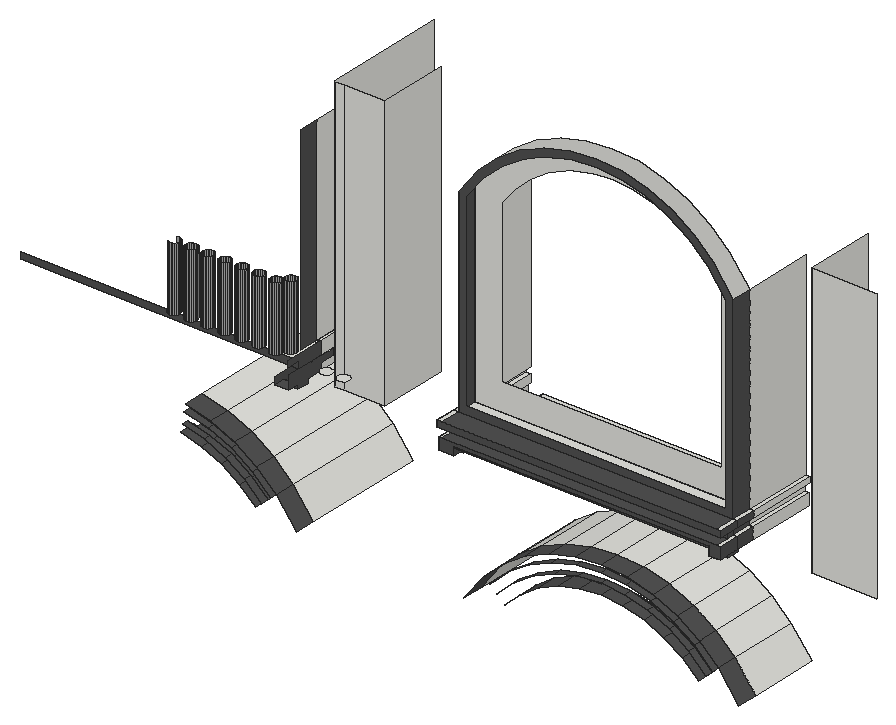
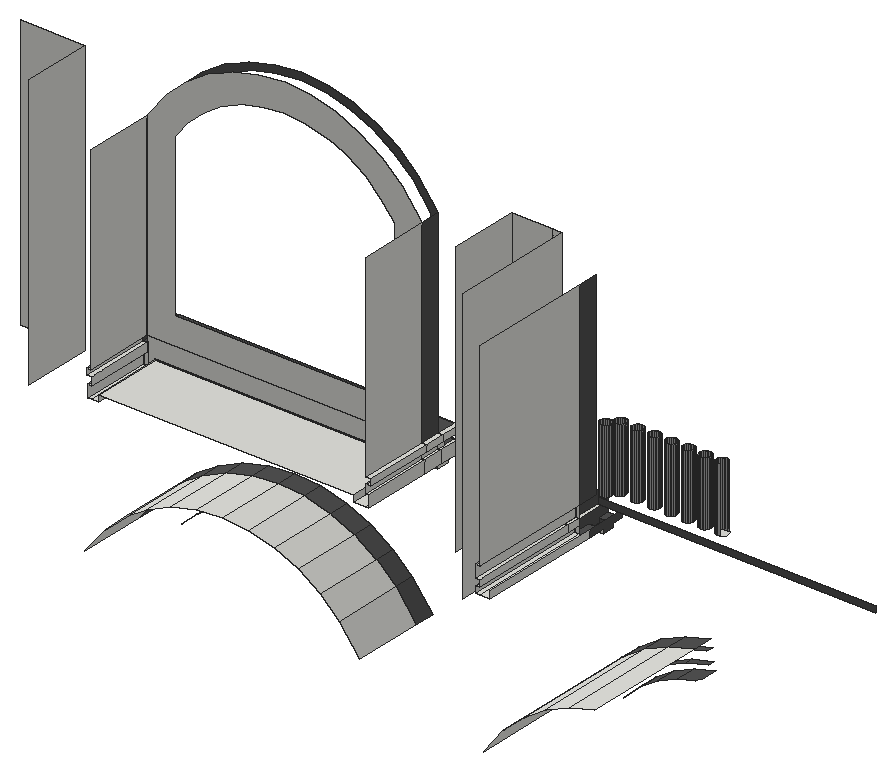
# SketchUp Ruby script. Lengths in inches.
U = 1.inch
M = Sketchup.active_model
def pt(a) = Geom::Point3d.new(a.map { |v| v * U })
def face(e, loops, mat)
  f = e.add_face(loops[0].map { |a| pt(a) })
  loops[1..].each { |l| e.add_face(l.map { |a| pt(a) }).erase! }
  f.material = f.back_material = mat if mat
  f
end
# faces: each face lists its corners as indices into pts; further lists are holes
def faces(e, pts, list, mat = nil) = list.each { |f| face(e, (f[0].is_a?(Array) ? f : [f]).map { |l| l.map { |i| pts[i] } }, mat) }
# xy, xz, yz: faces in a plane at the given z, y or x. An outline is a flat list of corners, or four numbers for a rectangle; further outlines are holes
def ring(l) = l.size == 4 ? [[l[0], l[1]], [l[2], l[1]], [l[2], l[3]], [l[0], l[3]]] : l.each_slice(2).to_a
def flat(e, list, mat, &to3) = list.each { |f| face(e, (f[0].is_a?(Array) ? f : [f]).map { |l| ring(l).map { |u, v| to3.(u, v) } }, mat) }
def xy(e, z, list, mat = nil) = flat(e, list, mat) { |x, y| [x, y, z] }
def xz(e, y, list, mat = nil) = flat(e, list, mat) { |x, z| [x, y, z] }
def yz(e, x, list, mat = nil) = flat(e, list, mat) { |y, z| [x, y, z] }
def lines(e, pts, list) = list.each { |a, b| e.add_line(pt(pts[a]), pt(pts[b])) }
# prism: a flat outline (further loops are holes) pulled along v
def prism(e, loops, v, mat = nil)
  f = face(e, loops, mat); d = Geom::Vector3d.new(v.map { |x| x * U })
  f.pushpull(f.normal.samedirection?(d) ? d.length : -d.length)
end
def box(e, o, s, mat = nil) = prism(e, [[o, [o[0] + s[0], o[1], o[2]], [o[0] + s[0], o[1] + s[1], o[2]], [o[0], o[1] + s[1], o[2]]]], [0, 0, s[2]], mat)
def at(x, y, z, deg = 0) = Geom::Transformation.translation(pt([x, y, z])) * Geom::Transformation.rotation(ORIGIN, Z_AXIS, deg.degrees)
def axes(o, x, y, z) = Geom::Transformation.new([*x, 0, *y, 0, *z, 0, *pt(o).to_a, 1])
def part(name) = M.definitions.add(name)
# library, detail: a bought-in or finely detailed component or shape, given as its bounding box
def library(name, o, s) = part(name).tap { |d| box(d.entities, o, s) }
def detail(e, o, s) = box(e.add_group.entities, o, s)
def put(e, d, t, mat = nil) = e.add_instance(d, t).tap { |i| i.material = mat if mat }
def group(e, t, mat = nil) = e.add_group.tap { |g| g.transformation = t; g.material = mat if mat }.entities
root = M.entities
M.materials.add("[0132_LightGray]").color = [169, 169, 169]
M.materials.add("[0135_DarkGray]").color = [81, 81, 81]
xy(root,482.35,[[358.5,36.95,364.76,42.1]],"[0135_DarkGray]")
xy(root,482.85,[[430.82,37.17,437.43,42.74]],"[0135_DarkGray]")
xy(root,483.16,[[549.38,35.78,554.39,41.4]],"[0135_DarkGray]")
xy(root,484.03,[[549.38,35.78,552.7,40.6875],[552.7,35.78,554.39,40.6875],[430.82,37.17,432.14,40.6875],[432.14,37.17,437.43,40.6875],[430.82,40.6875,432.14,42.74],
  [432.14,40.6875,437.43,42.74],[549.38,40.6875,552.7,41.4],[552.7,40.6875,554.39,41.4],[430.82,49.6875,432.14,80.4375],[432.14,49.6875,437.43,80.4375],
  [549.38,49.6875,552.7,80.4375],[552.7,49.6875,554.39,80.4375]])
xy(root,484.03,[[430.82,31.6875,432.14,37.17],[432.14,31.6875,437.43,37.17],[549.38,31.6875,552.7,35.78],[552.7,31.6875,554.39,35.78],[549.38,41.4,552.7,49.6875],
  [552.7,41.4,554.39,49.6875],[430.82,42.74,432.14,49.6875],[432.14,42.74,437.43,49.6875]],"[0135_DarkGray]")
xy(root,484.28,[[358.5,49.6875,363.14,104.375],[363.14,49.6875,364.76,104.375]])
xy(root,484.28,[[358.5,31.6875,364.76,36.95],[358.5,42.1,364.76,49.6875]],"[0135_DarkGray]")
xy(root,487.03,[[437.43,49.6875,549.38,80.4375]])
xy(root,487.03,[[437.43,31.6875,549.38,49.6875]],"[0135_DarkGray]")
xy(root,487.28,[[363.14,49.6875,364.76,55.75],[363.14,55.75,364.76,104.375]])
xy(root,487.72,[[437.43,31.6875,549.38,49.6875]])
xy(root,489.3125,[[430.82,31.6875,432.14,40.6875],[552.7,31.6875,554.39,40.6875],[430.82,40.6875,432.14,49.6875],[552.7,40.6875,554.39,49.6875],[430.82,49.6875,432.14,80.4375],
  [552.7,49.6875,554.39,80.4375]])
xy(root,489.3125,[[432.14,31.6875,552.7,37.6875]],"[0135_DarkGray]")
xy(root,490.18,[[363.14,37.6875,364.64,49.6875],[364.64,37.6875,364.76,55.75],[363.14,49.6875,364.64,55.75],[363.14,55.75,364.64,104.375]])
xy(root,492.99,[[430.01,49.6875,432.14,80.4375],[552.7,49.6875,554.64,80.4375]])
xy(root,492.99,[[430.01,31.6875,432.14,40.6875],[432.14,31.6875,552.7,37.6875],[552.7,31.6875,554.64,40.6875],[430.01,40.6875,432.14,49.6875],[552.7,40.6875,554.64,49.6875]],"[0135_DarkGray]")
xy(root,495.66,[[430.01,31.6875,432.14,40.6875],[552.82,31.6875,554.64,40.6875],[312.48,31.88,311.85,31.96,311.26,32.21,310.75,32.6,310.37,33.1,310.12,33.6875,310.04,34.32,310.12,34.95,310.37,35.54,310.75,36.04,311.26,36.43,311.85,36.67,312.48,36.76,313.11,36.67,313.7,36.43,314.2,36.04,314.59,35.54,314.83,34.95,314.91,34.32,314.83,33.6875,314.59,33.1,314.2,32.6,313.7,32.21,313.11,31.96],[319.91,31.88,319.28,31.96,318.7,32.21,318.19,32.6,317.8,33.1,317.56,33.6875,317.48,34.32,317.56,34.95,317.8,35.54,318.19,36.04,318.7,36.43,319.28,36.67,319.91,36.76,320.54,36.67,321.13,36.43,321.64,36.04,322.03,35.54,322.27,34.95,322.35,34.32,322.27,33.6875,322.03,33.1,321.64,32.6,321.13,32.21,320.54,31.96],[327.35,31.88,326.72,31.96,326.13,32.21,325.63,32.6,325.24,33.1,325,33.6875,324.91,34.32,325,34.95,325.24,35.54,325.63,36.04,326.13,36.43,326.72,36.67,327.35,36.76,327.98,36.67,328.57,36.43,329.08,36.04,329.46,35.54,329.71,34.95,329.79,34.32,329.71,33.6875,329.46,33.1,329.08,32.6,328.57,32.21,327.98,31.96],
  [334.79,31.88,334.16,31.96,333.57,32.21,333.07,32.6,332.68,33.1,332.43,33.6875,332.35,34.32,332.43,34.95,332.68,35.54,333.07,36.04,333.57,36.43,334.16,36.67,334.79,36.76,335.42,36.67,336.01,36.43,336.51,36.04,336.9,35.54,337.14,34.95,337.23,34.32,337.14,33.6875,336.9,33.1,336.51,32.6,336.01,32.21,335.42,31.96],[342.23,31.88,341.6,31.96,341.01,32.21,340.5,32.6,340.12,33.1,339.87,33.6875,339.79,34.32,339.87,34.95,340.12,35.54,340.5,36.04,341.01,36.43,341.6,36.67,342.23,36.76,342.86,36.67,343.45,36.43,343.95,36.04,344.34,35.54,344.58,34.95,344.66,34.32,344.58,33.6875,344.34,33.1,343.95,32.6,343.45,32.21,342.86,31.96],[349.66,31.88,349.03,31.96,348.45,32.21,347.94,32.6,347.55,33.1,347.31,33.6875,347.23,34.32,347.31,34.95,347.55,35.54,347.94,36.04,348.45,36.43,349.03,36.67,349.66,36.76,350.29,36.67,350.88,36.43,351.39,36.04,351.78,35.54,352.02,34.95,352.1,34.32,352.02,33.6875,351.78,33.1,351.39,32.6,350.88,32.21,350.29,31.96],[357.1,31.88,356.47,31.96,355.88,32.21,355.38,32.6,354.99,33.1,354.75,33.6875,354.66,34.32,354.75,34.95,354.99,35.54,355.38,36.04,355.88,36.43,356.47,36.67,357.1,36.76,357.73,36.67,358.32,36.43,358.83,36.04,359.21,35.54,359.46,34.95,359.54,34.32,359.46,33.6875,359.21,33.1,358.83,32.6,358.32,32.21,357.73,31.96],[379.41,31.88,380.04,31.96,380.63,32.21,381.14,32.6,381.53,33.1,381.77,33.6875,381.85,34.32,381.77,34.95,381.53,35.54,381.14,36.04,380.63,36.43,380.04,36.67,379.41,36.76,378.78,36.67,378.2,36.43,377.69,36.04,377.3,35.54,377.06,34.95,376.98,34.32,377.06,33.6875,377.3,33.1,377.69,32.6,378.2,32.21,378.78,31.96],
  [386.85,31.88,387.48,31.96,388.07,32.21,388.58,32.6,388.96,33.1,389.21,33.6875,389.29,34.32,389.21,34.95,388.96,35.54,388.58,36.04,388.07,36.43,387.48,36.67,386.85,36.76,386.22,36.67,385.63,36.43,385.13,36.04,384.74,35.54,384.5,34.95,384.41,34.32,384.5,33.6875,384.74,33.1,385.13,32.6,385.63,32.21,386.22,31.96],[360.59,35.72,359.96,35.81,359.37,36.05,358.86,36.4375,358.48,36.94,358.23,37.53,358.15,38.16,358.23,38.79,358.48,39.38,358.86,39.89,359.37,40.27,359.96,40.52,360.59,40.6,361.22,40.52,361.8,40.27,362.31,39.89,362.7,39.38,362.94,38.79,363.02,38.16,362.94,37.53,362.7,36.94,362.31,36.4375,361.8,36.05,361.22,35.81],[430.01,40.6875,432.14,49.6875],[432.14,40.6875,552.7,49.6875],[552.7,40.6875,552.82,49.6875],
  [552.82,40.6875,554.64,49.6875],[362.82,49.6875,363.14,104.375],[363.14,49.6875,364.64,104.375],[430.01,49.6875,432.14,80.4375],[552.82,49.6875,554.64,80.4375]])
xy(root,495.66,[[432.14,31.6875,552.82,40.6875]],"[0135_DarkGray]")
xz(root,31.6875,[[430.82,484.03,437.43,484.03,437.43,487.72,549.38,487.72,549.38,484.03,554.39,484.03,554.39,489.3125,430.82,489.3125],[437.43,487.03,549.38,487.72],[430.01,492.99,554.64,495.66]],"[0135_DarkGray]")
xz(root,35.78,[[549.38,483.16,554.39,484.03]],"[0135_DarkGray]")
xz(root,36.95,[[358.5,482.35,364.76,484.28]],"[0135_DarkGray]")
xz(root,37.17,[[430.82,482.85,437.43,484.03]],"[0135_DarkGray]")
xz(root,37.6875,[[432.14,489.3125,552.7,492.99],[242.14,490.18,364.64,493.07]],"[0135_DarkGray]")
xz(root,40.6875,[[[432.14,495.66,552.82,495.66,552.82,582.07,543.9,593.68,535.43,601.54,525.77,607.9,518.81,610.98,515.2,612.57,504,615.43,492.48,616.39,480.96,615.43,469.76,612.57,466.15,610.98,459.18,607.9,449.53,601.54,441.0625,593.68,432.14,582.07],[435.27,498.79,435.27,581.01,443.38,591.5625,451.47,599.07,460.6875,605.14,467.41,608.11,470.78,609.6,481.48,612.33,492.48,613.25,503.48,612.33,514.17,609.6,517.54,608.11,524.27,605.14,533.49,599.07,541.57,591.5625,549.69,581.01,549.69,498.79]]],"[0135_DarkGray]")
xz(root,41.4,[[549.38,483.16,554.39,484.03]])
xz(root,42.1,[[358.5,482.35,364.76,484.28]])
xz(root,42.74,[[430.82,482.85,437.43,484.03]],"[0135_DarkGray]")
xz(root,49.6875,[[370.55,480,370.74,600],[370.74,480,374.55,600],[374.55,480,392.7,600],[580.01,480,608.5,600],[430.82,484.03,432.14,489.3125],
  [432.14,484.03,437.43,484.03,437.43,487.72,549.38,487.72,549.38,484.03,552.7,484.03,552.7,495.66,432.14,495.66],[552.7,484.03,554.39,489.3125],[363.14,484.28,364.76,487.28],[437.43,487.03,549.38,487.72],[363.14,490.18,364.64,495.66],
  [[432.14,495.66,432.14,582.07,441.0625,593.68,449.53,601.54,459.18,607.9,466.15,610.98,469.76,612.57,480.96,615.43,492.48,616.39,504,615.43,515.2,612.57,518.81,610.98,525.77,607.9,535.43,601.54,543.9,593.68,552.82,582.07,552.82,495.66],[444.14,507.66,540.82,507.66,540.82,577.99,534.99,585.57,527.99,592.07,520.01,597.33,513.96,600,511.27,601.19,502,603.55,492.48,604.35,489.7,604.11,483.7,603.61,482.95,603.55,473.69,601.19,471,600,464.95,597.33,456.97,592.07,449.96,585.57,444.14,577.99]]])
xz(root,55.75,[[363.14,487.28,364.76,490.18]])
yz(root,358.5,[[49.6875,484.28,104.375,487.28]])
yz(root,358.5,[[36.95,482.35,36.95,484.28,31.6875,484.28,31.6875,487.28,49.6875,487.28,49.6875,484.28,42.1,484.28,42.1,482.35]],"[0135_DarkGray]")
yz(root,362.82,[[49.6875,495.66,104.375,582.07]])
yz(root,362.82,[[40.6875,495.66,49.6875,582.07]],"[0135_DarkGray]")
yz(root,363.14,[[49.6875,487.28,55.75,490.18],[55.75,487.28,104.375,490.18]])
yz(root,364.64,[[49.6875,490.18,104.375,495.66]])
yz(root,364.64,[[37.6875,490.18,49.6875,490.18,49.6875,495.66,31.6875,495.66,31.6875,493.07,37.6875,493.07]],"[0135_DarkGray]")
yz(root,364.76,[[49.6875,484.28,104.375,487.28]])
yz(root,364.76,[[36.95,482.35,42.1,482.35,42.1,484.28,49.6875,484.28,49.6875,487.28,55.75,487.28,55.75,490.18,31.6875,490.18,31.6875,484.28,36.95,484.28]],"[0135_DarkGray]")
yz(root,370.55,[[49.6875,480,104.375,600]])
yz(root,392.7,[[49.6875,480,80.4375,600]])
yz(root,430.01,[[31.6875,492.99,40.6875,495.66],[40.6875,492.99,49.6875,495.66],[49.6875,492.99,80.4375,495.66]])
yz(root,430.82,[[37.17,482.85,42.74,484.03],[31.6875,484.03,40.6875,489.3125],[40.6875,484.03,49.6875,489.3125],[49.6875,484.03,80.4375,489.3125]])
yz(root,432.14,[[37.6875,489.3125,40.6875,492.99],[40.6875,489.3125,49.6875,492.99],[49.6875,489.3125,80.4375,492.99],[49.6875,495.66,80.4375,582.07]])
yz(root,432.14,[[40.6875,495.66,49.6875,582.07]],"[0135_DarkGray]")
yz(root,437.43,[[49.6875,484.03,80.4375,487.03],[31.6875,487.03,40.6875,487.72],[40.6875,487.03,49.6875,487.72]])
yz(root,437.43,[[37.17,482.85,42.74,484.03],[31.6875,484.03,40.6875,487.03],[40.6875,484.03,49.6875,487.03]],"[0135_DarkGray]")
yz(root,549.38,[[49.6875,484.03,80.4375,487.03],[31.6875,487.03,40.6875,487.72],[40.6875,487.03,49.6875,487.72]])
yz(root,549.38,[[35.78,483.16,41.4,484.03],[31.6875,484.03,40.6875,487.03],[40.6875,484.03,49.6875,487.03]],"[0135_DarkGray]")
yz(root,552.7,[[49.6875,489.3125,80.4375,492.99]])
yz(root,552.7,[[37.6875,489.3125,40.6875,492.99],[40.6875,489.3125,49.6875,492.99]],"[0135_DarkGray]")
yz(root,552.82,[[49.6875,495.66,80.4375,582.07]])
yz(root,552.82,[[40.6875,495.66,49.6875,582.07]],"[0135_DarkGray]")
yz(root,554.39,[[49.6875,484.03,80.4375,489.3125]])
yz(root,554.39,[[35.78,483.16,41.4,484.03],[31.6875,484.03,40.6875,489.3125],[40.6875,484.03,49.6875,489.3125]],"[0135_DarkGray]")
yz(root,554.64,[[49.6875,492.99,80.4375,495.66]])
yz(root,554.64,[[31.6875,492.99,40.6875,495.66],[40.6875,492.99,49.6875,495.66]],"[0135_DarkGray]")
yz(root,580.01,[[49.6875,480,80.4375,600]])
p = [[361.14,49.6875,423.26],[352.21,49.6875,434.86],[352.21,40.6875,434.86],[361.14,40.6875,423.26],[434.7,49.6875,423.26],[443.625,49.6875,434.86],
  [443.625,40.6875,434.86],[434.7,40.6875,423.26],[546.46,49.6875,434.86],[555.39,49.6875,423.26],[555.39,40.6875,423.26],[546.46,40.6875,434.86],
  [352.21,104.375,434.86],[361.14,104.375,423.26],[434.7,80.4375,423.26],[443.625,80.4375,434.86],[546.46,80.4375,434.86],[555.39,80.4375,423.26],
  [336.3,49.6875,433.26],[343.31,49.6875,426.75],[343.31,40.6875,426.75],[336.3,40.6875,433.26],[452.53,49.6875,426.75],[459.53,49.6875,433.26],
  [459.53,40.6875,433.26],[452.53,40.6875,426.75],[530.55,49.6875,433.26],[537.56,49.6875,426.75],[537.56,40.6875,426.75],[530.55,40.6875,433.26],
  [345.9375,43.6875,429.15],[338.5,43.6875,436.06],[338.5,40.6875,436.06],[345.9375,40.6875,429.15],[456.63,43.6875,436.95],[449.06,43.6875,429.91],
  [449.06,40.6875,429.91],[456.63,40.6875,436.95],[541.02,43.6875,429.91],[533.45,43.6875,436.95],[533.45,40.6875,436.95],[541.02,40.6875,429.91],
  [341.7,43.6875,440.13],[349.77,43.6875,432.64],[349.77,40.6875,432.64],[341.7,40.6875,440.13],[445.98,43.6875,432.71],[454.0625,43.6875,440.22],
  [454.0625,40.6875,440.22],[445.98,40.6875,432.71],[536.02,43.6875,440.22],[544.1,43.6875,432.71],[544.1,40.6875,432.71],[536.02,40.6875,440.22],
  [328.32,49.6875,438.52],[328.32,40.6875,438.52],[467.51,49.6875,438.52],[467.51,40.6875,438.52],[522.57,49.6875,438.52],[522.57,40.6875,438.52],
  [343.74,49.6875,442.73],[343.74,40.6875,442.73],[452.09,49.6875,442.73],[452.09,40.6875,442.73],[537.99,49.6875,442.73],[537.99,40.6875,442.73],
  [343.74,104.375,442.73],[452.09,80.4375,442.73],[537.99,80.4375,442.73],[330.02,43.6875,441.64],[330.02,40.6875,441.64],[465.27,43.6875,442.63],
  [465.27,40.6875,442.63],[524.82,43.6875,442.63],[524.82,40.6875,442.63],[319.58,49.6875,442.38],[319.58,40.6875,442.38],[476.25,49.6875,442.38],
  [476.25,40.6875,442.38],[513.83,49.6875,442.38],[513.83,40.6875,442.38],[332.51,43.6875,446.1875],[332.51,40.6875,446.1875],[463.27,43.6875,446.29],
  [463.27,40.6875,446.29],[526.81,43.6875,446.29],[526.81,40.6875,446.29],[320.74,43.6875,445.74],[320.74,40.6875,445.74],[310.32,40.6875,444.74],
  [310.32,47.6875,444.74],[311.64,47.6875,444.4],[311.64,49.6875,444.4],[483.7,49.6875,444.27],[483.7,47.6875,444.27],[485.52,47.6875,444.74],
  [485.52,40.6875,444.74],[504.57,49.6875,444.74],[504.57,40.6875,444.74],[474.72,43.6875,446.81],[474.72,40.6875,446.81],[515.36,43.6875,446.81],
  [515.36,40.6875,446.81],[334.09,49.6875,449.09],[334.09,40.6875,449.09],[461.75,49.6875,449.09],[461.75,40.6875,449.09],[528.34,49.6875,449.09],
  [528.34,40.6875,449.09],[334.09,104.375,449.09],[461.75,80.4375,449.09],[528.34,80.4375,449.09],[485.52,49.6875,444.74],[489.7,47.6875,445.09],
  [489.7,49.6875,445.09],[495.04,49.6875,445.53],[495.04,40.6875,445.53],[310.91,43.6875,448.25],[310.91,40.6875,448.25],[322.43,43.6875,450.64],
  [322.43,40.6875,450.64],[473.36,43.6875,450.74],[473.36,40.6875,450.74],[516.72,43.6875,450.74],[516.72,40.6875,450.74],[484.74,43.6875,449.36],
  [484.74,40.6875,449.36],[505.34,43.6875,449.36],[505.34,40.6875,449.36],[323.51,49.6875,453.76],[323.51,40.6875,453.76],[472.32,49.6875,453.76],
  [472.32,40.6875,453.76],[517.76,49.6875,453.76],[517.76,40.6875,453.76],[323.51,104.375,453.76],[472.32,80.4375,453.76],[517.76,80.4375,453.76],
  [495.04,43.6875,450.22],[495.04,40.6875,450.22],[311.76,43.6875,453.36],[311.76,40.6875,453.36],[484.05,43.6875,453.47],[484.05,40.6875,453.47],
  [506.03,43.6875,453.47],[506.03,40.6875,453.47],[495.04,43.6875,454.38],[495.04,40.6875,454.38],[312.3125,49.6875,456.61],[312.3125,40.6875,456.61],
  [483.52,49.6875,456.61],[483.52,40.6875,456.61],[506.5625,49.6875,456.61],[506.5625,40.6875,456.61],[312.3125,104.375,456.61],[483.52,80.4375,456.61],
  [506.5625,80.4375,456.61],[495.04,49.6875,457.57],[495.04,40.6875,457.57],[495.04,80.4375,457.57],[311.85,31.96,495.66],[312.48,31.88,495.66],
  [312.48,31.88,523.91],[311.85,31.96,523.91],[313.11,31.96,495.66],[313.11,31.96,523.91],[319.28,31.96,495.66],[319.91,31.88,495.66],
  [319.91,31.88,523.91],[319.28,31.96,523.91],[320.54,31.96,495.66],[320.54,31.96,523.91],[326.72,31.96,495.66],[327.35,31.88,495.66],
  [327.35,31.88,523.91],[326.72,31.96,523.91],[327.98,31.96,495.66],[327.98,31.96,523.91],[334.16,31.96,495.66],[334.79,31.88,495.66],
  [334.79,31.88,523.91],[334.16,31.96,523.91],[335.42,31.96,495.66],[335.42,31.96,523.91],[341.6,31.96,495.66],[342.23,31.88,495.66],
  [342.23,31.88,523.91],[341.6,31.96,523.91],[342.86,31.96,495.66],[342.86,31.96,523.91],[349.03,31.96,495.66],[349.66,31.88,495.66],
  [349.66,31.88,523.91],[349.03,31.96,523.91],[350.29,31.96,495.66],[350.29,31.96,523.91],[356.47,31.96,495.66],[357.1,31.88,495.66],
  [357.1,31.88,523.91],[356.47,31.96,523.91],[357.73,31.96,495.66],[357.73,31.96,523.91],[311.26,32.21,495.66],[311.26,32.21,523.91],
  [313.7,32.21,495.66],[313.7,32.21,523.91],[318.7,32.21,495.66],[318.7,32.21,523.91],[321.13,32.21,495.66],[321.13,32.21,523.91],
  [326.13,32.21,495.66],[326.13,32.21,523.91],[328.57,32.21,495.66],[328.57,32.21,523.91],[333.57,32.21,495.66],[333.57,32.21,523.91],
  [336.01,32.21,495.66],[336.01,32.21,523.91],[341.01,32.21,495.66],[341.01,32.21,523.91],[343.45,32.21,495.66],[343.45,32.21,523.91],
  [348.45,32.21,495.66],[348.45,32.21,523.91],[350.88,32.21,495.66],[350.88,32.21,523.91],[355.88,32.21,495.66],[355.88,32.21,523.91],
  [358.32,32.21,495.66],[358.32,32.21,523.91],[314.2,32.6,495.66],[314.2,32.6,523.91],[318.19,32.6,495.66],[318.19,32.6,523.91],
  [321.64,32.6,495.66],[321.64,32.6,523.91],[325.63,32.6,495.66],[325.63,32.6,523.91],[329.08,32.6,495.66],[329.08,32.6,523.91],
  [333.07,32.6,495.66],[333.07,32.6,523.91],[336.51,32.6,495.66],[336.51,32.6,523.91],[340.5,32.6,495.66],[340.5,32.6,523.91],
  [343.95,32.6,495.66],[343.95,32.6,523.91],[347.94,32.6,495.66],[347.94,32.6,523.91],[351.39,32.6,495.66],[351.39,32.6,523.91],
  [355.38,32.6,495.66],[355.38,32.6,523.91],[358.83,32.6,495.66],[358.83,32.6,523.91],[314.59,33.1,495.66],[314.59,33.1,523.91],
  [317.8,33.1,495.66],[317.8,33.1,523.91],[322.03,33.1,495.66],[322.03,33.1,523.91],[325.24,33.1,495.66],[325.24,33.1,523.91],
  [329.46,33.1,495.66],[329.46,33.1,523.91],[332.68,33.1,495.66],[332.68,33.1,523.91],[336.9,33.1,495.66],[336.9,33.1,523.91],
  [340.12,33.1,495.66],[340.12,33.1,523.91],[344.34,33.1,495.66],[344.34,33.1,523.91],[347.55,33.1,495.66],[347.55,33.1,523.91],
  [351.78,33.1,495.66],[351.78,33.1,523.91],[354.99,33.1,495.66],[354.99,33.1,523.91],[359.21,33.1,495.66],[359.21,33.1,523.91],
  [314.83,33.6875,495.66],[314.83,33.6875,523.91],[317.56,33.6875,495.66],[317.56,33.6875,523.91],[322.27,33.6875,495.66],[322.27,33.6875,523.91],
  [325,33.6875,495.66],[325,33.6875,523.91],[329.71,33.6875,495.66],[329.71,33.6875,523.91],[332.43,33.6875,495.66],[332.43,33.6875,523.91],
  [337.14,33.6875,495.66],[337.14,33.6875,523.91],[339.87,33.6875,495.66],[339.87,33.6875,523.91],[344.58,33.6875,495.66],[344.58,33.6875,523.91],
  [347.31,33.6875,495.66],[347.31,33.6875,523.91],[352.02,33.6875,495.66],[352.02,33.6875,523.91],[354.75,33.6875,495.66],[354.75,33.6875,523.91],
  [359.46,33.6875,495.66],[359.46,33.6875,523.91],[314.91,34.32,495.66],[314.91,34.32,523.91],[317.48,34.32,495.66],[317.48,34.32,523.91],
  [322.35,34.32,495.66],[322.35,34.32,523.91],[324.91,34.32,495.66],[324.91,34.32,523.91],[329.79,34.32,495.66],[329.79,34.32,523.91],
  [332.35,34.32,495.66],[332.35,34.32,523.91],[337.23,34.32,495.66],[337.23,34.32,523.91],[339.79,34.32,495.66],[339.79,34.32,523.91],
  [344.66,34.32,495.66],[344.66,34.32,523.91],[347.23,34.32,495.66],[347.23,34.32,523.91],[352.1,34.32,495.66],[352.1,34.32,523.91],
  [354.66,34.32,495.66],[354.66,34.32,523.91],[359.54,34.32,495.66],[359.54,34.32,523.91],[314.83,34.95,495.66],[314.83,34.95,523.91],
  [317.56,34.95,495.66],[317.56,34.95,523.91],[322.27,34.95,495.66],[322.27,34.95,523.91],[325,34.95,495.66],[325,34.95,523.91],
  [329.71,34.95,495.66],[329.71,34.95,523.91],[332.43,34.95,495.66],[332.43,34.95,523.91],[337.14,34.95,495.66],[337.14,34.95,523.91],
  [339.87,34.95,495.66],[339.87,34.95,523.91],[344.58,34.95,495.66],[344.58,34.95,523.91],[347.31,34.95,495.66],[347.31,34.95,523.91],
  [352.02,34.95,495.66],[352.02,34.95,523.91],[354.75,34.95,495.66],[354.75,34.95,523.91],[359.46,34.95,495.66],[359.46,34.95,523.91],
  [314.59,35.54,495.66],[314.59,35.54,523.91],[317.8,35.54,495.66],[317.8,35.54,523.91],[322.03,35.54,495.66],[322.03,35.54,523.91],
  [325.24,35.54,495.66],[325.24,35.54,523.91],[329.46,35.54,495.66],[329.46,35.54,523.91],[332.68,35.54,495.66],[332.68,35.54,523.91],
  [336.9,35.54,495.66],[336.9,35.54,523.91],[340.12,35.54,495.66],[340.12,35.54,523.91],[344.34,35.54,495.66],[344.34,35.54,523.91],
  [347.55,35.54,495.66],[347.55,35.54,523.91],[351.78,35.54,495.66],[351.78,35.54,523.91],[354.99,35.54,495.66],[354.99,35.54,523.91],
  [359.21,35.54,495.66],[359.21,35.54,523.91],[314.2,36.04,495.66],[314.2,36.04,523.91],[318.19,36.04,495.66],[318.19,36.04,523.91],
  [321.64,36.04,495.66],[321.64,36.04,523.91],[325.63,36.04,495.66],[325.63,36.04,523.91],[329.08,36.04,495.66],[329.08,36.04,523.91],
  [333.07,36.04,495.66],[333.07,36.04,523.91],[336.51,36.04,495.66],[336.51,36.04,523.91],[340.5,36.04,495.66],[340.5,36.04,523.91],
  [343.95,36.04,495.66],[343.95,36.04,523.91],[347.94,36.04,495.66],[347.94,36.04,523.91],[351.39,36.04,495.66],[351.39,36.04,523.91],
  [355.38,36.04,495.66],[355.38,36.04,523.91],[358.83,36.04,495.66],[358.83,36.04,523.91],[359.96,35.81,495.66],[360.59,35.72,495.66],
  [360.59,35.72,523.91],[359.96,35.81,523.91],[361.22,35.81,495.66],[361.22,35.81,523.91],[359.37,36.05,495.66],[359.37,36.05,523.91],
  [361.8,36.05,495.66],[361.8,36.05,523.91],[313.7,36.43,495.66],[313.7,36.43,523.91],[318.7,36.43,495.66],[318.7,36.43,523.91],
  [321.13,36.43,495.66],[321.13,36.43,523.91],[326.13,36.43,495.66],[326.13,36.43,523.91],[328.57,36.43,495.66],[328.57,36.43,523.91],
  [333.57,36.43,495.66],[333.57,36.43,523.91],[336.01,36.43,495.66],[336.01,36.43,523.91],[341.01,36.43,495.66],[341.01,36.43,523.91],
  [343.45,36.43,495.66],[343.45,36.43,523.91],[348.45,36.43,495.66],[348.45,36.43,523.91],[350.88,36.43,495.66],[350.88,36.43,523.91],
  [355.88,36.43,495.66],[355.88,36.43,523.91],[358.32,36.43,495.66],[358.32,36.43,523.91],[358.86,36.4375,495.66],[358.86,36.4375,523.91],
  [362.31,36.4375,495.66],[362.31,36.4375,523.91],[313.11,36.67,495.66],[313.11,36.67,523.91],[319.28,36.67,495.66],[319.28,36.67,523.91],
  [320.54,36.67,495.66],[320.54,36.67,523.91],[326.72,36.67,495.66],[326.72,36.67,523.91],[327.98,36.67,495.66],[327.98,36.67,523.91],
  [334.16,36.67,495.66],[334.16,36.67,523.91],[335.42,36.67,495.66],[335.42,36.67,523.91],[341.6,36.67,495.66],[341.6,36.67,523.91],
  [342.86,36.67,495.66],[342.86,36.67,523.91],[349.03,36.67,495.66],[349.03,36.67,523.91],[350.29,36.67,495.66],[350.29,36.67,523.91],
  [356.47,36.67,495.66],[356.47,36.67,523.91],[357.73,36.67,495.66],[357.73,36.67,523.91],[358.48,36.94,495.66],[358.48,36.94,523.91],
  [362.7,36.94,495.66],[362.7,36.94,523.91],[312.48,36.76,495.66],[311.85,36.67,495.66],[311.85,36.67,523.91],[312.48,36.76,523.91],
  [319.91,36.76,495.66],[319.91,36.76,523.91],[327.35,36.76,495.66],[327.35,36.76,523.91],[334.79,36.76,495.66],[334.79,36.76,523.91],
  [342.23,36.76,495.66],[342.23,36.76,523.91],[349.66,36.76,495.66],[349.66,36.76,523.91],[357.1,36.76,495.66],[357.1,36.76,523.91],
  [358.23,37.53,495.66],[358.23,37.53,523.91],[362.94,37.53,495.66],[362.94,37.53,523.91],[358.15,38.16,495.66],[358.15,38.16,523.91],
  [363.02,38.16,495.66],[363.02,38.16,523.91],[358.23,38.79,495.66],[358.23,38.79,523.91],[362.94,38.79,495.66],[362.94,38.79,523.91],
  [358.48,39.38,495.66],[358.48,39.38,523.91],[362.7,39.38,495.66],[362.7,39.38,523.91],[358.86,39.89,495.66],[358.86,39.89,523.91],
  [362.31,39.89,495.66],[362.31,39.89,523.91],[359.37,40.27,495.66],[359.37,40.27,523.91],[361.8,40.27,495.66],[361.8,40.27,523.91],
  [359.96,40.52,495.66],[359.96,40.52,523.91],[361.22,40.52,495.66],[361.22,40.52,523.91],[360.59,40.6,495.66],[360.59,40.6,523.91],
  [363.14,37.6875,490.18],[363.14,37.6875,487.28],[432.14,37.6875,492.99],[432.14,37.6875,495.66],[432.14,37.6875,487.03],[432.14,37.6875,489.3125]]
faces(root,p,[[0,1,2,3],[4,5,6,7],[8,9,10,11],[18,19,20,21],[22,23,24,25],[26,27,28,29],[30,31,32,33],[34,35,36,37],
  [38,39,40,41],[42,43,44,45],[46,47,48,49],[50,51,52,53],[54,18,21,55],[23,56,57,24],[58,26,29,59],[1,60,61,2],
  [5,62,63,6],[64,8,11,65],[31,69,70,32],[71,34,37,72],[39,73,74,40],[75,54,55,76],[56,77,78,57],[79,58,59,80],
  [81,42,45,82],[47,83,84,48],[85,50,53,86],[69,87,88,70],[89,90,91,92,75,76],[77,93,94,95,96,78],[97,79,80,98],[99,71,72,100],
  [73,101,102,74],[60,103,104,61],[62,105,106,63],[107,64,65,108],[96,95,113,114,115,116],[115,97,98,116],[87,117,118,88],[119,81,82,120],
  [83,121,122,84],[123,85,86,124],[125,99,100,126],[101,127,128,102],[103,129,130,104],[105,131,132,106],[133,107,108,134],[138,125,126,139],
  [127,138,139,128],[140,119,120,141],[121,142,143,122],[144,123,124,145],[142,146,147,143],[146,144,145,147],[129,148,149,130],[131,150,151,132],
  [152,133,134,153],[150,157,158,151],[157,152,153,158]],"[0135_DarkGray]")
faces(root,p,[[0,1,12,13],[5,4,14,15],[9,8,16,17],[1,60,66,12],[62,5,15,67],[8,64,68,16],[60,103,109,66],[105,62,67,110],
  [64,107,111,68],[93,112,95,94],[112,114,113,95],[103,129,135,109],[131,105,110,136],[107,133,137,111],[129,148,154,135],[150,131,136,155],
  [133,152,156,137],[157,150,155,159],[152,157,159,156]])
faces(root,p,[[160,161,162,163],[161,164,165,162],[166,167,168,169],[167,170,171,168],[172,173,174,175],[173,176,177,174],[178,179,180,181],[179,182,183,180],
  [184,185,186,187],[185,188,189,186],[190,191,192,193],[191,194,195,192],[196,197,198,199],[197,200,201,198],[202,160,163,203],[164,204,205,165],
  [206,166,169,207],[170,208,209,171],[210,172,175,211],[176,212,213,177],[214,178,181,215],[182,216,217,183],[218,184,187,219],[188,220,221,189],
  [222,190,193,223],[194,224,225,195],[226,196,199,227],[200,228,229,201],[204,230,231,205],[232,206,207,233],[208,234,235,209],[236,210,211,237],
  [212,238,239,213],[240,214,215,241],[216,242,243,217],[244,218,219,245],[220,246,247,221],[248,222,223,249],[224,250,251,225],[252,226,227,253],
  [228,254,255,229],[230,256,257,231],[258,232,233,259],[234,260,261,235],[262,236,237,263],[238,264,265,239],[266,240,241,267],[242,268,269,243],
  [270,244,245,271],[246,272,273,247],[274,248,249,275],[250,276,277,251],[278,252,253,279],[254,280,281,255],[256,282,283,257],[284,258,259,285],
  [260,286,287,261],[288,262,263,289],[264,290,291,265],[292,266,267,293],[268,294,295,269],[296,270,271,297],[272,298,299,273],[300,274,275,301],
  [276,302,303,277],[304,278,279,305],[280,306,307,281],[282,308,309,283],[310,284,285,311],[286,312,313,287],[314,288,289,315],[290,316,317,291],
  [318,292,293,319],[294,320,321,295],[322,296,297,323],[298,324,325,299],[326,300,301,327],[302,328,329,303],[330,304,305,331],[306,332,333,307],
  [308,334,335,309],[336,310,311,337],[312,338,339,313],[340,314,315,341],[316,342,343,317],[344,318,319,345],[320,346,347,321],[348,322,323,349],
  [324,350,351,325],[352,326,327,353],[328,354,355,329],[356,330,331,357],[332,358,359,333],[334,360,361,335],[362,336,337,363],[338,364,365,339],
  [366,340,341,367],[342,368,369,343],[370,344,345,371],[346,372,373,347],[374,348,349,375],[350,376,377,351],[378,352,353,379],[354,380,381,355],
  [382,356,357,383],[358,384,385,359],[360,386,387,361],[388,362,363,389],[364,390,391,365],[392,366,367,393],[368,394,395,369],[396,370,371,397],
  [372,398,399,373],[400,374,375,401],[376,402,403,377],[404,378,379,405],[380,406,407,381],[408,382,383,409],[384,410,411,385],[412,413,414,415],
  [413,416,417,414],[418,412,415,419],[416,420,421,417],[386,422,423,387],[424,388,389,425],[390,426,427,391],[428,392,393,429],[394,430,431,395],
  [432,396,397,433],[398,434,435,399],[436,400,401,437],[402,438,439,403],[440,404,405,441],[406,442,443,407],[444,408,409,445],[410,446,447,411],
  [448,418,419,449],[420,450,451,421],[422,452,453,423],[454,424,425,455],[426,456,457,427],[458,428,429,459],[430,460,461,431],[462,432,433,463],
  [434,464,465,435],[466,436,437,467],[438,468,469,439],[470,440,441,471],[442,472,473,443],[474,444,445,475],[446,476,477,447],[478,448,449,479],
  [450,480,481,451],[482,483,484,485],[452,482,485,453],[486,454,455,487],[456,486,487,457],[488,458,459,489],[460,488,489,461],[490,462,463,491],
  [464,490,491,465],[492,466,467,493],[468,492,493,469],[494,470,471,495],[472,494,495,473],[496,474,475,497],[476,496,497,477],[498,478,479,499],
  [480,500,501,481],[502,498,499,503],[500,504,505,501],[506,502,503,507],[504,508,509,505],[510,506,507,511],[508,512,513,509],[514,510,511,515],
  [512,516,517,513],[518,514,515,519],[516,520,521,517],[522,518,519,523],[520,524,525,521],[526,522,523,527],[524,526,527,525]],"[0132_LightGray]")
lines(root,p,[[528,529],[530,531],[532,533]])
